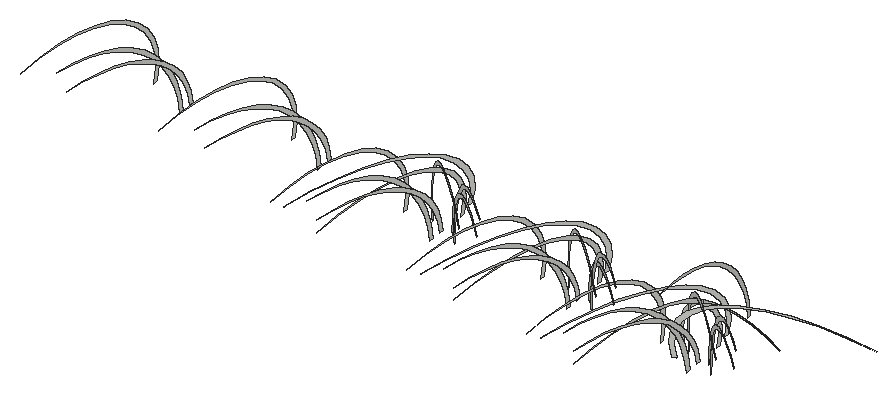
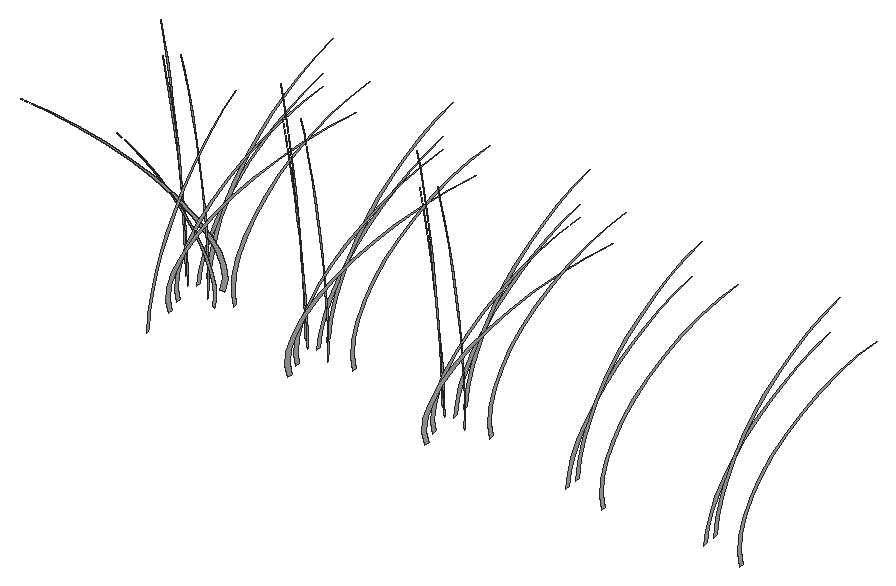
# SketchUp Ruby script. Lengths in inches.
U = 1.inch
M = Sketchup.active_model
def pt(a) = Geom::Point3d.new(a.map { |v| v * U })
def face(e, loops, mat)
  f = e.add_face(loops[0].map { |a| pt(a) })
  loops[1..].each { |l| e.add_face(l.map { |a| pt(a) }).erase! }
  f.material = f.back_material = mat if mat
  f
end
# faces: each face lists its corners as indices into pts; further lists are holes
def faces(e, pts, list, mat = nil) = list.each { |f| face(e, (f[0].is_a?(Array) ? f : [f]).map { |l| l.map { |i| pts[i] } }, mat) }
# xy, xz, yz: faces in a plane at the given z, y or x. An outline is a flat list of corners, or four numbers for a rectangle; further outlines are holes
def ring(l) = l.size == 4 ? [[l[0], l[1]], [l[2], l[1]], [l[2], l[3]], [l[0], l[3]]] : l.each_slice(2).to_a
def flat(e, list, mat, &to3) = list.each { |f| face(e, (f[0].is_a?(Array) ? f : [f]).map { |l| ring(l).map { |u, v| to3.(u, v) } }, mat) }
def xy(e, z, list, mat = nil) = flat(e, list, mat) { |x, y| [x, y, z] }
def xz(e, y, list, mat = nil) = flat(e, list, mat) { |x, z| [x, y, z] }
def yz(e, x, list, mat = nil) = flat(e, list, mat) { |y, z| [x, y, z] }
def lines(e, pts, list) = list.each { |a, b| e.add_line(pt(pts[a]), pt(pts[b])) }
# prism: a flat outline (further loops are holes) pulled along v
def prism(e, loops, v, mat = nil)
  f = face(e, loops, mat); d = Geom::Vector3d.new(v.map { |x| x * U })
  f.pushpull(f.normal.samedirection?(d) ? d.length : -d.length)
end
def box(e, o, s, mat = nil) = prism(e, [[o, [o[0] + s[0], o[1], o[2]], [o[0] + s[0], o[1] + s[1], o[2]], [o[0], o[1] + s[1], o[2]]]], [0, 0, s[2]], mat)
def at(x, y, z, deg = 0) = Geom::Transformation.translation(pt([x, y, z])) * Geom::Transformation.rotation(ORIGIN, Z_AXIS, deg.degrees)
def axes(o, x, y, z) = Geom::Transformation.new([*x, 0, *y, 0, *z, 0, *pt(o).to_a, 1])
def part(name) = M.definitions.add(name)
# library, detail: a bought-in or finely detailed component or shape, given as its bounding box
def library(name, o, s) = part(name).tap { |d| box(d.entities, o, s) }
def detail(e, o, s) = box(e.add_group.entities, o, s)
def put(e, d, t, mat = nil) = e.add_instance(d, t).tap { |i| i.material = mat if mat }
def group(e, t, mat = nil) = e.add_group.tap { |g| g.transformation = t; g.material = mat if mat }.entities
root = M.entities
g1 = group(root,at(379.95,269.61,0))
p = [[0.12,-0.92,0],[0.05,-0.41,0],[0,0,1.75],[0.02,-0.16,3.51],[0.11,-0.9,5.24],[0.27,-2.18,6.89],
  [0.5,-3.98,8.42],[0.79,-6.26,9.8],[1.13,-8.95,10.98],[1.51,-12,11.95],[1.93,-15.32,12.67],[2.37,-18.83,13.13],
  [2.83,-22.45,13.32],[3.28,-26.08,13.23],[2.84,-22.52,13.25],[2.39,-18.99,13],[1.96,-15.57,12.5],[1.56,-12.36,11.75],
  [1.19,-9.41,10.78],[0.86,-6.8,9.6],[0.58,-4.59,8.25],[0.36,-2.83,6.75],[0.2,-1.56,5.13],[0.1,-0.81,3.44],
  [0.07,-0.59,1.72]]
faces(g1,p,[[0,1,2,3,4,5,6,7,8,9,10,11,12,13,14,15,16,17,18,19,20,21,22,23,24]])
g2 = group(root,at(385.49,268.11,0))
p = [[2.6,-20.61,12.375],[2.99,-23.72,12.7],[2.61,-20.71,12.31],[2.24,-17.8,11.76],[1.89,-15.03,11.07],[1.56,-12.42,10.23],
  [1.26,-10.01,9.27],[0.99,-7.82,8.2],[0.74,-5.88,7.01],[0.53,-4.21,5.74],[0.36,-2.83,4.38],[0.22,-1.74,2.96],
  [0.125,-0.98,1.5],[0.07,-0.54,0],[0,0,0],[0.05,-0.36,1.53],[0.14,-1.08,3.03],[0.27,-2.14,4.49],
  [0.45,-3.54,5.875],[0.66,-5.24,7.18],[0.91,-7.24,8.375],[1.2,-9.51,9.46],[1.51,-12.01,10.41],[1.85,-14.72,11.22],
  [2.22,-17.6,11.88]]
faces(g2,p,[[0,1,2,3,4,5,6,7,8,9,10,11,12,13,14,15,16,17,18,19,20,21,22,23,24]])
g3 = group(root,at(385.73,266.2,0))
p = [[2.6,-20.61,15.34],[2.99,-23.72,15.75],[2.61,-20.71,15.26],[2.24,-17.8,14.58],[1.89,-15.03,13.72],[1.56,-12.42,12.69],
  [1.26,-10.01,11.5],[0.99,-7.82,10.16],[0.74,-5.88,8.7],[0.53,-4.21,7.11],[0.36,-2.83,5.43],[0.22,-1.74,3.67],
  [0.125,-0.98,1.86],[0.07,-0.54,0],[0,0,0],[0.05,-0.36,1.9],[0.14,-1.08,3.76],[0.27,-2.14,5.57],
  [0.45,-3.54,7.28],[0.66,-5.24,8.9],[0.91,-7.24,10.39],[1.2,-9.51,11.73],[1.51,-12.01,12.91],[1.85,-14.72,13.91],
  [2.22,-17.6,14.73]]
faces(g3,p,[[0,1,2,3,4,5,6,7,8,9,10,11,12,13,14,15,16,17,18,19,20,21,22,23,24]])
g4 = group(root,at(397.81,269.19,0))
p = [[0.12,-0.92,0],[0.05,-0.41,0],[0,0,1.75],[0.02,-0.16,3.51],[0.11,-0.9,5.24],[0.27,-2.18,6.89],
  [0.5,-3.98,8.42],[0.79,-6.26,9.8],[1.13,-8.95,10.98],[1.51,-12,11.95],[1.93,-15.32,12.67],[2.37,-18.83,13.13],
  [2.83,-22.45,13.32],[3.28,-26.08,13.23],[2.84,-22.52,13.25],[2.39,-18.99,13],[1.96,-15.57,12.5],[1.56,-12.36,11.75],
  [1.19,-9.41,10.78],[0.86,-6.8,9.6],[0.58,-4.59,8.25],[0.36,-2.83,6.75],[0.2,-1.56,5.13],[0.1,-0.81,3.44],
  [0.07,-0.59,1.72]]
faces(g4,p,[[0,1,2,3,4,5,6,7,8,9,10,11,12,13,14,15,16,17,18,19,20,21,22,23,24]])
g5 = group(root,at(403.35,267.7,0))
p = [[2.6,-20.61,12.375],[2.99,-23.72,12.7],[2.61,-20.71,12.31],[2.24,-17.8,11.76],[1.89,-15.03,11.07],[1.56,-12.42,10.23],
  [1.26,-10.01,9.27],[0.99,-7.82,8.2],[0.74,-5.88,7.01],[0.53,-4.21,5.74],[0.36,-2.83,4.38],[0.22,-1.74,2.96],
  [0.125,-0.98,1.5],[0.07,-0.54,0],[0,0,0],[0.05,-0.36,1.53],[0.14,-1.08,3.03],[0.27,-2.14,4.49],
  [0.45,-3.54,5.875],[0.66,-5.24,7.18],[0.91,-7.24,8.375],[1.2,-9.51,9.46],[1.51,-12.01,10.41],[1.85,-14.72,11.22],
  [2.22,-17.6,11.88]]
faces(g5,p,[[0,1,2,3,4,5,6,7,8,9,10,11,12,13,14,15,16,17,18,19,20,21,22,23,24]])
g6 = group(root,at(403.59,265.78,0))
p = [[2.6,-20.61,15.34],[2.99,-23.72,15.75],[2.61,-20.71,15.26],[2.24,-17.8,14.58],[1.89,-15.03,13.72],[1.56,-12.42,12.69],
  [1.26,-10.01,11.5],[0.99,-7.82,10.16],[0.74,-5.88,8.7],[0.53,-4.21,7.11],[0.36,-2.83,5.43],[0.22,-1.74,3.67],
  [0.125,-0.98,1.86],[0.07,-0.54,0],[0,0,0],[0.05,-0.36,1.9],[0.14,-1.08,3.76],[0.27,-2.14,5.57],
  [0.45,-3.54,7.28],[0.66,-5.24,8.9],[0.91,-7.24,10.39],[1.2,-9.51,11.73],[1.51,-12.01,12.91],[1.85,-14.72,13.91],
  [2.22,-17.6,14.73]]
faces(g6,p,[[0,1,2,3,4,5,6,7,8,9,10,11,12,13,14,15,16,17,18,19,20,21,22,23,24]])
g7 = group(root,at(415.52,264.84,0))
p = [[0.12,-0.92,0],[0.05,-0.41,0],[0,0,1.75],[0.02,-0.16,3.51],[0.11,-0.9,5.24],[0.27,-2.18,6.89],
  [0.5,-3.98,8.42],[0.79,-6.26,9.8],[1.13,-8.95,10.98],[1.51,-12,11.95],[1.93,-15.32,12.67],[2.37,-18.83,13.13],
  [2.83,-22.45,13.32],[3.28,-26.08,13.23],[2.84,-22.52,13.25],[2.39,-18.99,13],[1.96,-15.57,12.5],[1.56,-12.36,11.75],
  [1.19,-9.41,10.78],[0.86,-6.8,9.6],[0.58,-4.59,8.25],[0.36,-2.83,6.75],[0.2,-1.56,5.13],[0.1,-0.81,3.44],
  [0.07,-0.59,1.72]]
faces(g7,p,[[0,1,2,3,4,5,6,7,8,9,10,11,12,13,14,15,16,17,18,19,20,21,22,23,24]])
g8 = group(root,at(419.86,269.87,0))
p = [[-0.06,-0.99,0],[-0.03,-0.44,0],[0,0,1.49],[-0.01,-0.18,2.99],[-0.06,-0.97,4.45],[-0.14,-2.36,5.86],
  [-0.26,-4.3,7.16],[-0.4,-6.76,8.33],[-0.58,-9.67,9.33],[-0.77,-12.96,10.15],[-0.99,-16.54,10.77],[-1.22,-20.34,11.16],
  [-1.45,-24.24,11.32],[-1.68,-28.17,11.24],[-1.45,-24.32,11.26],[-1.23,-20.51,11.05],[-1.01,-16.82,10.625],[-0.8,-13.35,9.99],
  [-0.61,-10.16,9.16],[-0.4375,-7.35,8.16],[-0.3,-4.96,7.01],[-0.18,-3.06,5.73],[-0.1,-1.69,4.36],[-0.05,-0.87,2.93],
  [-0.04,-0.64,1.46]]
faces(g8,p,[[0,1,2,3,4,5,6,7,8,9,10,11,12,13,14,15,16,17,18,19,20,21,22,23,24]])
g9 = group(root,at(420.52,267.62,0))
p = [[0.125,-0.99,0],[0.06,-0.4375,0],[0,0,1.49],[0.02,-0.18,2.99],[0.12,-0.96,4.45],[0.3,-2.34,5.86],
  [0.54,-4.28,7.16],[0.85,-6.72,8.33],[1.21,-9.61,9.33],[1.62,-12.88,10.15],[2.07,-16.44,10.77],[2.55,-20.21,11.16],
  [3.03,-24.1,11.32],[3.53,-28,11.24],[3.04,-24.17,11.26],[2.57,-20.38,11.05],[2.11,-16.72,10.625],[1.67,-13.27,9.99],
  [1.27,-10.1,9.16],[0.92,-7.3,8.16],[0.62,-4.93,7.01],[0.38,-3.04,5.73],[0.21,-1.67,4.36],[0.11,-0.87,2.93],
  [0.08,-0.64,1.46]]
faces(g9,p,[[0,1,2,3,4,5,6,7,8,9,10,11,12,13,14,15,16,17,18,19,20,21,22,23,24]])
g10 = group(root,at(421.06,263.35,0))
p = [[2.6,-20.61,12.375],[2.99,-23.72,12.7],[2.61,-20.71,12.31],[2.24,-17.8,11.76],[1.89,-15.03,11.07],[1.56,-12.42,10.23],
  [1.26,-10.01,9.27],[0.99,-7.82,8.2],[0.74,-5.88,7.01],[0.53,-4.21,5.74],[0.36,-2.83,4.38],[0.22,-1.74,2.96],
  [0.125,-0.98,1.5],[0.07,-0.54,0],[0,0,0],[0.05,-0.36,1.53],[0.14,-1.08,3.03],[0.27,-2.14,4.49],
  [0.45,-3.54,5.875],[0.66,-5.24,7.18],[0.91,-7.24,8.375],[1.2,-9.51,9.46],[1.51,-12.01,10.41],[1.85,-14.72,11.22],
  [2.22,-17.6,11.88]]
faces(g10,p,[[0,1,2,3,4,5,6,7,8,9,10,11,12,13,14,15,16,17,18,19,20,21,22,23,24]])
g11 = group(root,at(421.3,261.43,0))
p = [[2.6,-20.61,15.34],[2.99,-23.72,15.75],[2.61,-20.71,15.26],[2.24,-17.8,14.58],[1.89,-15.03,13.72],[1.56,-12.42,12.69],
  [1.26,-10.01,11.5],[0.99,-7.82,10.16],[0.74,-5.88,8.7],[0.53,-4.21,7.11],[0.36,-2.83,5.43],[0.22,-1.74,3.67],
  [0.125,-0.98,1.86],[0.07,-0.54,0],[0,0,0],[0.05,-0.36,1.9],[0.14,-1.08,3.76],[0.27,-2.14,5.57],
  [0.45,-3.54,7.28],[0.66,-5.24,8.9],[0.91,-7.24,10.39],[1.2,-9.51,11.73],[1.51,-12.01,12.91],[1.85,-14.72,13.91],
  [2.22,-17.6,14.73]]
faces(g11,p,[[0,1,2,3,4,5,6,7,8,9,10,11,12,13,14,15,16,17,18,19,20,21,22,23,24]])
g12 = group(root,at(418.3125,264.93,0))
p = [[0.65,-0.66,0],[0.29,-0.29,0],[0,0,1.75],[0.12,-0.12,3.51],[0.64,-0.64,5.24],[1.55,-1.5625,6.89],
  [2.82,-2.86,8.42],[4.4375,-4.49,9.8],[6.35,-6.42,10.98],[8.5,-8.6,11.95],[10.85,-10.98,12.67],[13.34,-13.49,13.13],
  [15.91,-16.09,13.32],[18.48,-18.69,13.23],[15.96,-16.14,13.25],[13.45,-13.61,13],[11.04,-11.16,12.5],[8.76,-8.86,11.75],
  [6.67,-6.74,10.78],[4.82,-4.875,9.6],[3.25,-3.29,8.25],[2.01,-2.03,6.75],[1.11,-1.12,5.13],[0.57,-0.58,3.44],
  [0.42,-0.42,1.72]]
faces(g12,p,[[0,1,2,3,4,5,6,7,8,9,10,11,12,13,14,15,16,17,18,19,20,21,22,23,24]])
g13 = group(root,at(421.83,263.8,0))
p = [[14.61,-14.77,12.375],[16.8125,-17,12.7],[14.68,-14.84,12.31],[12.62,-12.76,11.76],[10.65,-10.77,11.07],[8.8,-8.9,10.23],
  [7.09,-7.17,9.27],[5.54,-5.61,8.2],[4.17,-4.22,7.01],[2.98,-3.02,5.74],[2,-2.02,4.38],[1.24,-1.25,2.96],
  [0.69,-0.7,1.5],[0.38,-0.38,0],[0,0,0],[0.26,-0.26,1.53],[0.77,-0.77,3.03],[1.52,-1.54,4.49],
  [2.51,-2.53,5.875],[3.72,-3.76,7.18],[5.13,-5.19,8.375],[6.74,-6.8125,9.46],[8.51,-8.61,10.41],[10.43,-10.55,11.22],
  [12.47,-12.61,11.88]]
faces(g13,p,[[0,1,2,3,4,5,6,7,8,9,10,11,12,13,14,15,16,17,18,19,20,21,22,23,24]])
g14 = group(root,at(423.19,262.43,0))
p = [[14.61,-14.77,15.34],[16.8125,-17,15.75],[14.68,-14.84,15.26],[12.62,-12.76,14.58],[10.65,-10.77,13.72],[8.8,-8.9,12.69],
  [7.09,-7.17,11.5],[5.54,-5.61,10.16],[4.17,-4.22,8.7],[2.98,-3.02,7.11],[2,-2.02,5.43],[1.24,-1.25,3.67],
  [0.69,-0.7,1.86],[0.38,-0.38,0],[0,0,0],[0.26,-0.26,1.9],[0.77,-0.77,3.76],[1.52,-1.54,5.57],
  [2.51,-2.53,7.28],[3.72,-3.76,8.9],[5.13,-5.19,10.39],[6.74,-6.8125,11.73],[8.51,-8.61,12.91],[10.43,-10.55,13.91],
  [12.47,-12.61,14.73]]
faces(g14,p,[[0,1,2,3,4,5,6,7,8,9,10,11,12,13,14,15,16,17,18,19,20,21,22,23,24]])
g15 = group(root,at(434.67,262.625,0))
p = [[0.12,-0.92,0],[0.05,-0.41,0],[0,0,1.75],[0.02,-0.16,3.51],[0.11,-0.9,5.24],[0.27,-2.18,6.89],
  [0.5,-3.98,8.42],[0.79,-6.26,9.8],[1.13,-8.95,10.98],[1.51,-12,11.95],[1.93,-15.32,12.67],[2.37,-18.83,13.13],
  [2.83,-22.45,13.32],[3.28,-26.08,13.23],[2.84,-22.52,13.25],[2.39,-18.99,13],[1.96,-15.57,12.5],[1.56,-12.36,11.75],
  [1.19,-9.41,10.78],[0.86,-6.8,9.6],[0.58,-4.59,8.25],[0.36,-2.83,6.75],[0.2,-1.56,5.13],[0.1,-0.81,3.44],
  [0.07,-0.59,1.72]]
faces(g15,p,[[0,1,2,3,4,5,6,7,8,9,10,11,12,13,14,15,16,17,18,19,20,21,22,23,24]])
g16 = group(root,at(439.01,267.66,0))
p = [[-0.06,-0.99,0],[-0.03,-0.44,0],[0,0,1.49],[-0.01,-0.18,2.99],[-0.06,-0.97,4.45],[-0.14,-2.36,5.86],
  [-0.26,-4.3,7.16],[-0.4,-6.76,8.33],[-0.58,-9.67,9.33],[-0.77,-12.96,10.15],[-0.99,-16.54,10.77],[-1.22,-20.34,11.16],
  [-1.45,-24.24,11.32],[-1.68,-28.17,11.24],[-1.45,-24.32,11.26],[-1.23,-20.51,11.05],[-1.01,-16.82,10.625],[-0.8,-13.35,9.99],
  [-0.61,-10.16,9.16],[-0.4375,-7.35,8.16],[-0.3,-4.96,7.01],[-0.18,-3.06,5.73],[-0.1,-1.69,4.36],[-0.05,-0.87,2.93],
  [-0.04,-0.64,1.46]]
faces(g16,p,[[0,1,2,3,4,5,6,7,8,9,10,11,12,13,14,15,16,17,18,19,20,21,22,23,24]])
g17 = group(root,at(439.67,265.41,0))
p = [[0.125,-0.99,0],[0.06,-0.4375,0],[0,0,1.49],[0.02,-0.18,2.99],[0.12,-0.96,4.45],[0.3,-2.34,5.86],
  [0.54,-4.28,7.16],[0.85,-6.72,8.33],[1.21,-9.61,9.33],[1.62,-12.88,10.15],[2.07,-16.44,10.77],[2.55,-20.21,11.16],
  [3.03,-24.1,11.32],[3.53,-28,11.24],[3.04,-24.17,11.26],[2.57,-20.38,11.05],[2.11,-16.72,10.625],[1.67,-13.27,9.99],
  [1.27,-10.1,9.16],[0.92,-7.3,8.16],[0.62,-4.93,7.01],[0.38,-3.04,5.73],[0.21,-1.67,4.36],[0.11,-0.87,2.93],
  [0.08,-0.64,1.46]]
faces(g17,p,[[0,1,2,3,4,5,6,7,8,9,10,11,12,13,14,15,16,17,18,19,20,21,22,23,24]])
g18 = group(root,at(440.21,261.13,0))
p = [[2.6,-20.61,12.375],[2.99,-23.72,12.7],[2.61,-20.71,12.31],[2.24,-17.8,11.76],[1.89,-15.03,11.07],[1.56,-12.42,10.23],
  [1.26,-10.01,9.27],[0.99,-7.82,8.2],[0.74,-5.88,7.01],[0.53,-4.21,5.74],[0.36,-2.83,4.38],[0.22,-1.74,2.96],
  [0.125,-0.98,1.5],[0.07,-0.54,0],[0,0,0],[0.05,-0.36,1.53],[0.14,-1.08,3.03],[0.27,-2.14,4.49],
  [0.45,-3.54,5.875],[0.66,-5.24,7.18],[0.91,-7.24,8.375],[1.2,-9.51,9.46],[1.51,-12.01,10.41],[1.85,-14.72,11.22],
  [2.22,-17.6,11.88]]
faces(g18,p,[[0,1,2,3,4,5,6,7,8,9,10,11,12,13,14,15,16,17,18,19,20,21,22,23,24]])
g19 = group(root,at(440.45,259.22,0))
p = [[2.6,-20.61,15.34],[2.99,-23.72,15.75],[2.61,-20.71,15.26],[2.24,-17.8,14.58],[1.89,-15.03,13.72],[1.56,-12.42,12.69],
  [1.26,-10.01,11.5],[0.99,-7.82,10.16],[0.74,-5.88,8.7],[0.53,-4.21,7.11],[0.36,-2.83,5.43],[0.22,-1.74,3.67],
  [0.125,-0.98,1.86],[0.07,-0.54,0],[0,0,0],[0.05,-0.36,1.9],[0.14,-1.08,3.76],[0.27,-2.14,5.57],
  [0.45,-3.54,7.28],[0.66,-5.24,8.9],[0.91,-7.24,10.39],[1.2,-9.51,11.73],[1.51,-12.01,12.91],[1.85,-14.72,13.91],
  [2.22,-17.6,14.73]]
faces(g19,p,[[0,1,2,3,4,5,6,7,8,9,10,11,12,13,14,15,16,17,18,19,20,21,22,23,24]])
g20 = group(root,at(437.46,262.72,0))
p = [[0.65,-0.66,0],[0.29,-0.29,0],[0,0,1.75],[0.12,-0.12,3.51],[0.64,-0.64,5.24],[1.55,-1.5625,6.89],
  [2.82,-2.86,8.42],[4.4375,-4.49,9.8],[6.35,-6.42,10.98],[8.5,-8.6,11.95],[10.85,-10.98,12.67],[13.34,-13.49,13.13],
  [15.91,-16.09,13.32],[18.48,-18.69,13.23],[15.96,-16.14,13.25],[13.45,-13.61,13],[11.04,-11.16,12.5],[8.76,-8.86,11.75],
  [6.67,-6.74,10.78],[4.82,-4.875,9.6],[3.25,-3.29,8.25],[2.01,-2.03,6.75],[1.11,-1.12,5.13],[0.57,-0.58,3.44],
  [0.42,-0.42,1.72]]
faces(g20,p,[[0,1,2,3,4,5,6,7,8,9,10,11,12,13,14,15,16,17,18,19,20,21,22,23,24]])
g21 = group(root,at(440.98,261.59,0))
p = [[14.61,-14.77,12.375],[16.8125,-17,12.7],[14.68,-14.84,12.31],[12.62,-12.76,11.76],[10.65,-10.77,11.07],[8.8,-8.9,10.23],
  [7.09,-7.17,9.27],[5.54,-5.61,8.2],[4.17,-4.22,7.01],[2.98,-3.02,5.74],[2,-2.02,4.38],[1.24,-1.25,2.96],
  [0.69,-0.7,1.5],[0.38,-0.38,0],[0,0,0],[0.26,-0.26,1.53],[0.77,-0.77,3.03],[1.52,-1.54,4.49],
  [2.51,-2.53,5.875],[3.72,-3.76,7.18],[5.13,-5.19,8.375],[6.74,-6.8125,9.46],[8.51,-8.61,10.41],[10.43,-10.55,11.22],
  [12.47,-12.61,11.88]]
faces(g21,p,[[0,1,2,3,4,5,6,7,8,9,10,11,12,13,14,15,16,17,18,19,20,21,22,23,24]])
g22 = group(root,at(442.34,260.21,0))
p = [[14.61,-14.77,15.34],[16.8125,-17,15.75],[14.68,-14.84,15.26],[12.62,-12.76,14.58],[10.65,-10.77,13.72],[8.8,-8.9,12.69],
  [7.09,-7.17,11.5],[5.54,-5.61,10.16],[4.17,-4.22,8.7],[2.98,-3.02,7.11],[2,-2.02,5.43],[1.24,-1.25,3.67],
  [0.69,-0.7,1.86],[0.38,-0.38,0],[0,0,0],[0.26,-0.26,1.9],[0.77,-0.77,3.76],[1.52,-1.54,5.57],
  [2.51,-2.53,7.28],[3.72,-3.76,8.9],[5.13,-5.19,10.39],[6.74,-6.8125,11.73],[8.51,-8.61,12.91],[10.43,-10.55,13.91],
  [12.47,-12.61,14.73]]
faces(g22,p,[[0,1,2,3,4,5,6,7,8,9,10,11,12,13,14,15,16,17,18,19,20,21,22,23,24]])
g23 = group(root,at(451.98,259.97,0))
p = [[0.12,-0.92,0],[0.05,-0.41,0],[0,0,1.75],[0.02,-0.16,3.51],[0.11,-0.9,5.24],[0.27,-2.18,6.89],
  [0.5,-3.98,8.42],[0.79,-6.26,9.8],[1.13,-8.95,10.98],[1.51,-12,11.95],[1.93,-15.32,12.67],[2.37,-18.83,13.13],
  [2.83,-22.45,13.32],[3.28,-26.08,13.23],[2.84,-22.52,13.25],[2.39,-18.99,13],[1.96,-15.57,12.5],[1.56,-12.36,11.75],
  [1.19,-9.41,10.78],[0.86,-6.8,9.6],[0.58,-4.59,8.25],[0.36,-2.83,6.75],[0.2,-1.56,5.13],[0.1,-0.81,3.44],
  [0.07,-0.59,1.72]]
faces(g23,p,[[0,1,2,3,4,5,6,7,8,9,10,11,12,13,14,15,16,17,18,19,20,21,22,23,24]])
g24 = group(root,at(456.33,265,0))
p = [[-0.06,-0.99,0],[-0.03,-0.44,0],[0,0,1.49],[-0.01,-0.18,2.99],[-0.06,-0.97,4.45],[-0.14,-2.36,5.86],
  [-0.26,-4.3,7.16],[-0.4,-6.76,8.33],[-0.58,-9.67,9.33],[-0.77,-12.96,10.15],[-0.99,-16.54,10.77],[-1.22,-20.34,11.16],
  [-1.45,-24.24,11.32],[-1.68,-28.17,11.24],[-1.45,-24.32,11.26],[-1.23,-20.51,11.05],[-1.01,-16.82,10.625],[-0.8,-13.35,9.99],
  [-0.61,-10.16,9.16],[-0.4375,-7.35,8.16],[-0.3,-4.96,7.01],[-0.18,-3.06,5.73],[-0.1,-1.69,4.36],[-0.05,-0.87,2.93],
  [-0.04,-0.64,1.46]]
faces(g24,p,[[0,1,2,3,4,5,6,7,8,9,10,11,12,13,14,15,16,17,18,19,20,21,22,23,24]])
g25 = group(root,at(456.98,262.75,0))
p = [[0.125,-0.99,0],[0.06,-0.4375,0],[0,0,1.49],[0.02,-0.18,2.99],[0.12,-0.96,4.45],[0.3,-2.34,5.86],
  [0.54,-4.28,7.16],[0.85,-6.72,8.33],[1.21,-9.61,9.33],[1.62,-12.88,10.15],[2.07,-16.44,10.77],[2.55,-20.21,11.16],
  [3.03,-24.1,11.32],[3.53,-28,11.24],[3.04,-24.17,11.26],[2.57,-20.38,11.05],[2.11,-16.72,10.625],[1.67,-13.27,9.99],
  [1.27,-10.1,9.16],[0.92,-7.3,8.16],[0.62,-4.93,7.01],[0.38,-3.04,5.73],[0.21,-1.67,4.36],[0.11,-0.87,2.93],
  [0.08,-0.64,1.46]]
faces(g25,p,[[0,1,2,3,4,5,6,7,8,9,10,11,12,13,14,15,16,17,18,19,20,21,22,23,24]])
g26 = group(root,at(457.52,258.48,0))
p = [[2.6,-20.61,12.375],[2.99,-23.72,12.7],[2.61,-20.71,12.31],[2.24,-17.8,11.76],[1.89,-15.03,11.07],[1.56,-12.42,10.23],
  [1.26,-10.01,9.27],[0.99,-7.82,8.2],[0.74,-5.88,7.01],[0.53,-4.21,5.74],[0.36,-2.83,4.38],[0.22,-1.74,2.96],
  [0.125,-0.98,1.5],[0.07,-0.54,0],[0,0,0],[0.05,-0.36,1.53],[0.14,-1.08,3.03],[0.27,-2.14,4.49],
  [0.45,-3.54,5.875],[0.66,-5.24,7.18],[0.91,-7.24,8.375],[1.2,-9.51,9.46],[1.51,-12.01,10.41],[1.85,-14.72,11.22],
  [2.22,-17.6,11.88]]
faces(g26,p,[[0,1,2,3,4,5,6,7,8,9,10,11,12,13,14,15,16,17,18,19,20,21,22,23,24]])
g27 = group(root,at(455.58,268.94,0))
p = [[6.07,-19.87,14.56],[6.99,-22.87,14.94],[6.1,-19.96,14.48],[5.25,-17.16,13.83],[4.43,-14.49,13.02],[3.66,-11.97,12.04],
  [2.95,-9.65,10.91],[2.31,-7.54,9.64],[1.73,-5.67,8.25],[1.24,-4.06,6.75],[0.83,-2.72,5.15],[0.51,-1.68,3.49],
  [0.29,-0.94,1.76],[0.16,-0.52,0],[0,0,0],[0.11,-0.35,1.8],[0.32,-1.04,3.57],[0.63,-2.07,5.28],
  [1.04,-3.41,6.91],[1.55,-5.05,8.44],[2.13,-6.98,9.85],[2.8,-9.16,11.13],[3.54,-11.58,12.25],[4.34,-14.1875,13.2],
  [5.1875,-16.96,13.97]]
faces(g27,p,[[0,1,2,3,4,5,6,7,8,9,10,11,12,13,14,15,16,17,18,19,20,21,22,23,24]])
g28 = group(root,at(457.76,256.5625,0))
p = [[2.6,-20.61,15.34],[2.99,-23.72,15.75],[2.61,-20.71,15.26],[2.24,-17.8,14.58],[1.89,-15.03,13.72],[1.56,-12.42,12.69],
  [1.26,-10.01,11.5],[0.99,-7.82,10.16],[0.74,-5.88,8.7],[0.53,-4.21,7.11],[0.36,-2.83,5.43],[0.22,-1.74,3.67],
  [0.125,-0.98,1.86],[0.07,-0.54,0],[0,0,0],[0.05,-0.36,1.9],[0.14,-1.08,3.76],[0.27,-2.14,5.57],
  [0.45,-3.54,7.28],[0.66,-5.24,8.9],[0.91,-7.24,10.39],[1.2,-9.51,11.73],[1.51,-12.01,12.91],[1.85,-14.72,13.91],
  [2.22,-17.6,14.73]]
faces(g28,p,[[0,1,2,3,4,5,6,7,8,9,10,11,12,13,14,15,16,17,18,19,20,21,22,23,24]])
g29 = group(root,at(453.07,261.02,0))
p = [[0.69,-0.31,0],[0.31,-0.14,0],[0,0,1.24],[0.125,-0.06,2.49],[0.68,-0.3,3.72],[1.65,-0.73,4.89],
  [3.01,-1.34,5.98],[4.73,-2.11,6.95],[6.76,-3.01,7.8],[9.06,-4.04,8.48],[11.5625,-5.15,8.99],[14.21,-6.33,9.32],
  [16.94,-7.55,9.46],[19.6875,-8.77,9.39],[17,-7.58,9.4],[14.33,-6.39,9.23],[11.76,-5.24,8.875],[9.33,-4.16,8.35],
  [7.1,-3.17,7.65],[5.14,-2.29,6.82],[3.47,-1.55,5.86],[2.14,-0.95,4.79],[1.18,-0.52,3.64],[0.61,-0.27,2.45],
  [0.45,-0.2,1.22]]
faces(g29,p,[[0,1,2,3,4,5,6,7,8,9,10,11,12,13,14,15,16,17,18,19,20,21,22,23,24]])
g30 = group(root,at(454.78,260.0625,0))
p = [[0.65,-0.66,0],[0.29,-0.29,0],[0,0,1.75],[0.12,-0.12,3.51],[0.64,-0.64,5.24],[1.55,-1.5625,6.89],
  [2.82,-2.86,8.42],[4.4375,-4.49,9.8],[6.35,-6.42,10.98],[8.5,-8.6,11.95],[10.85,-10.98,12.67],[13.34,-13.49,13.13],
  [15.91,-16.09,13.32],[18.48,-18.69,13.23],[15.96,-16.14,13.25],[13.45,-13.61,13],[11.04,-11.16,12.5],[8.76,-8.86,11.75],
  [6.67,-6.74,10.78],[4.82,-4.875,9.6],[3.25,-3.29,8.25],[2.01,-2.03,6.75],[1.11,-1.12,5.13],[0.57,-0.58,3.44],
  [0.42,-0.42,1.72]]
faces(g30,p,[[0,1,2,3,4,5,6,7,8,9,10,11,12,13,14,15,16,17,18,19,20,21,22,23,24]])
g31 = group(root,at(458.29,258.93,0))
p = [[14.61,-14.77,12.375],[16.8125,-17,12.7],[14.68,-14.84,12.31],[12.62,-12.76,11.76],[10.65,-10.77,11.07],[8.8,-8.9,10.23],
  [7.09,-7.17,9.27],[5.54,-5.61,8.2],[4.17,-4.22,7.01],[2.98,-3.02,5.74],[2,-2.02,4.38],[1.24,-1.25,2.96],
  [0.69,-0.7,1.5],[0.38,-0.38,0],[0,0,0],[0.26,-0.26,1.53],[0.77,-0.77,3.03],[1.52,-1.54,4.49],
  [2.51,-2.53,5.875],[3.72,-3.76,7.18],[5.13,-5.19,8.375],[6.74,-6.8125,9.46],[8.51,-8.61,10.41],[10.43,-10.55,11.22],
  [12.47,-12.61,11.88]]
faces(g31,p,[[0,1,2,3,4,5,6,7,8,9,10,11,12,13,14,15,16,17,18,19,20,21,22,23,24]])
g32 = group(root,at(459.65,257.5625,0))
p = [[14.61,-14.77,15.34],[16.8125,-17,15.75],[14.68,-14.84,15.26],[12.62,-12.76,14.58],[10.65,-10.77,13.72],[8.8,-8.9,12.69],
  [7.09,-7.17,11.5],[5.54,-5.61,10.16],[4.17,-4.22,8.7],[2.98,-3.02,7.11],[2,-2.02,5.43],[1.24,-1.25,3.67],
  [0.69,-0.7,1.86],[0.38,-0.38,0],[0,0,0],[0.26,-0.26,1.9],[0.77,-0.77,3.76],[1.52,-1.54,5.57],
  [2.51,-2.53,7.28],[3.72,-3.76,8.9],[5.13,-5.19,10.39],[6.74,-6.8125,11.73],[8.51,-8.61,12.91],[10.43,-10.55,13.91],
  [12.47,-12.61,14.73]]
faces(g32,p,[[0,1,2,3,4,5,6,7,8,9,10,11,12,13,14,15,16,17,18,19,20,21,22,23,24]])
g33 = group(root,at(454.26,257.72,0))
p = [[0.99,-0.08,0],[0.44,-0.04,0],[0,0,1.49],[0.18,-0.01,2.99],[0.97,-0.08,4.45],[2.35,-0.19,5.86],
  [4.3,-0.35,7.16],[6.75,-0.55,8.33],[9.66,-0.78,9.33],[12.9375,-1.05,10.15],[16.52,-1.34,10.77],[20.31,-1.64,11.16],
  [24.21,-1.96,11.32],[28.13,-2.27,11.24],[24.28,-1.96,11.26],[20.48,-1.66,11.05],[16.8,-1.36,10.625],[13.33,-1.08,9.99],
  [10.15,-0.82,9.16],[7.34,-0.59,8.16],[4.95,-0.4,7.01],[3.05,-0.25,5.73],[1.68,-0.14,4.36],[0.87,-0.07,2.93],
  [0.64,-0.05,1.46]]
faces(g33,p,[[0,1,2,3,4,5,6,7,8,9,10,11,12,13,14,15,16,17,18,19,20,21,22,23,24]])
